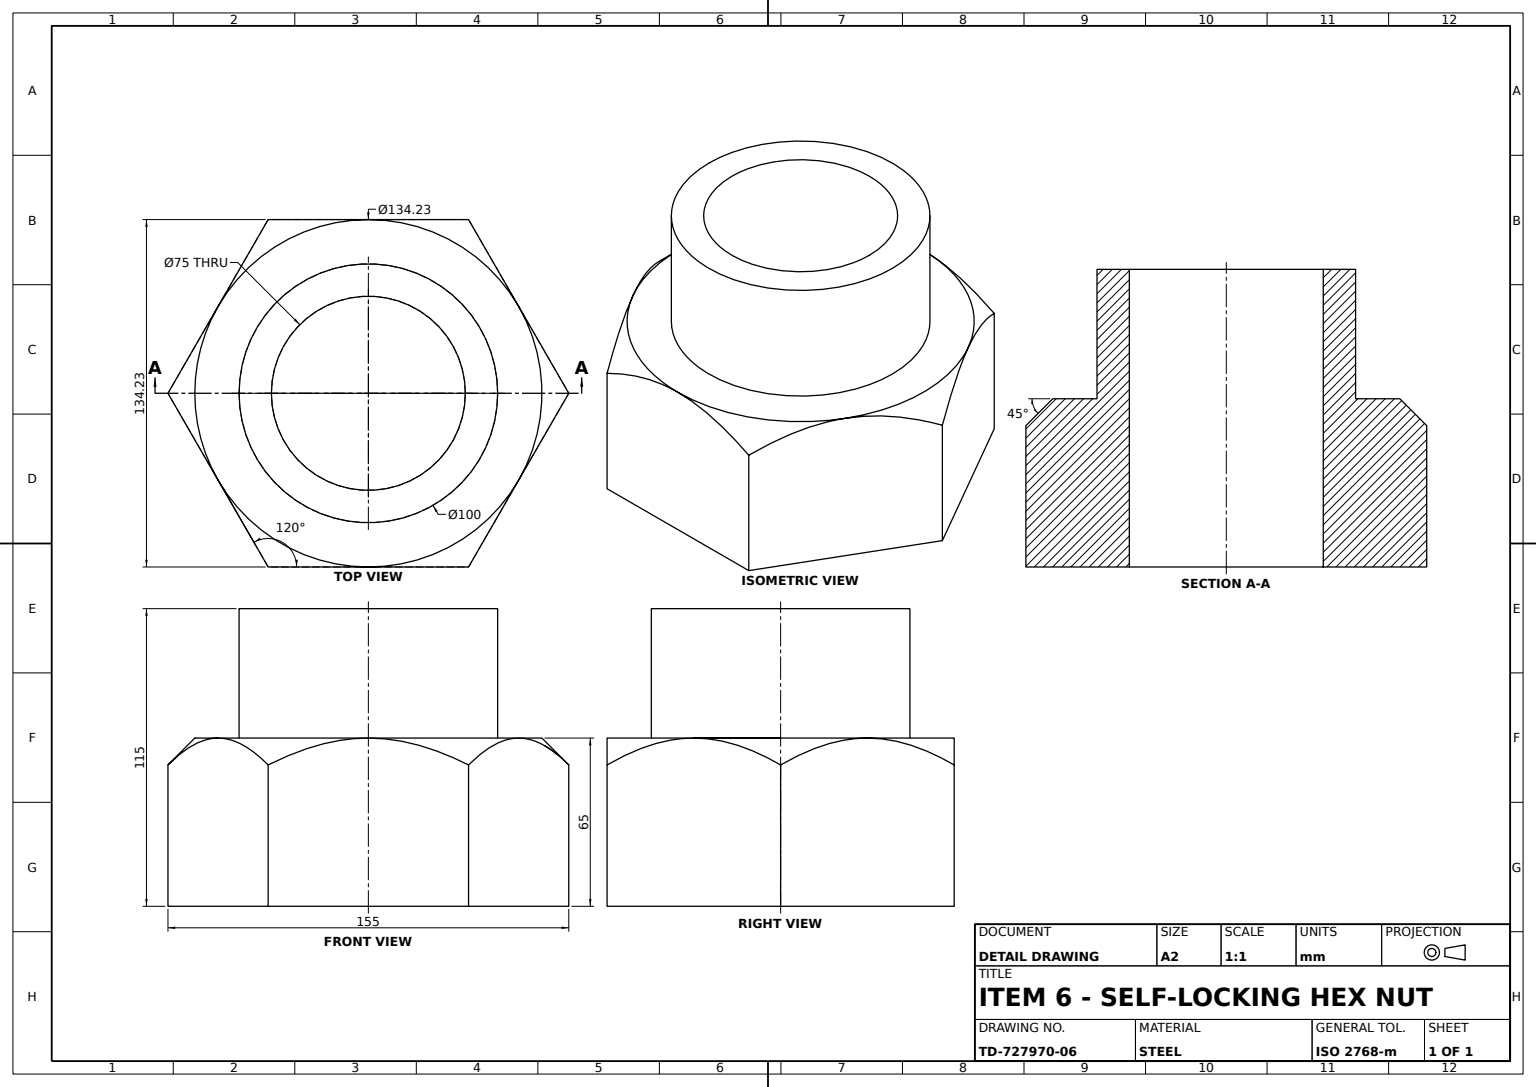
ISO-10303-21;
HEADER;
FILE_DESCRIPTION((''),'2;1');
FILE_NAME('','',(''),(''),'','','');
FILE_SCHEMA(('AUTOMOTIVE_DESIGN'));
ENDSEC;
DATA;
#1=APPLICATION_CONTEXT('');
#2=PRODUCT_CONTEXT('',#1,'mechanical');
#3=PRODUCT('','','',(#2));
#4=PRODUCT_DEFINITION_FORMATION('','',#3);
#5=PRODUCT_DEFINITION_CONTEXT('',#1,'design');
#6=PRODUCT_DEFINITION('','',#4,#5);
#7=PRODUCT_DEFINITION_SHAPE('','',#6);
#8=(LENGTH_UNIT()NAMED_UNIT(*)SI_UNIT(.MILLI.,.METRE.));
#9=(NAMED_UNIT(*)PLANE_ANGLE_UNIT()SI_UNIT($,.RADIAN.));
#10=(NAMED_UNIT(*)SI_UNIT($,.STERADIAN.)SOLID_ANGLE_UNIT());
#11=UNCERTAINTY_MEASURE_WITH_UNIT(LENGTH_MEASURE(1.E-05),#8,'distance_accuracy_value','');
#12=(GEOMETRIC_REPRESENTATION_CONTEXT(3)GLOBAL_UNCERTAINTY_ASSIGNED_CONTEXT((#11))GLOBAL_UNIT_ASSIGNED_CONTEXT((#8,#9,#10))REPRESENTATION_CONTEXT('',''));
#13=CARTESIAN_POINT('',(67.116969,54.616969,38.75));
#14=VERTEX_POINT('',#13);
#15=CARTESIAN_POINT('',(67.116969,0.,38.75));
#16=VERTEX_POINT('',#15);
#17=CARTESIAN_POINT('',(67.116969,65.,38.75));
#18=DIRECTION('',(0.,-1.,0.));
#19=VECTOR('',#18,1000.);
#20=LINE('',#17,#19);
#21=EDGE_CURVE('',#14,#16,#20,.T.);
#22=ORIENTED_EDGE('',*,*,#21,.F.);
#23=CARTESIAN_POINT('',(33.558484,65.,58.125));
#24=VERTEX_POINT('',#23);
#25=CARTESIAN_POINT('',(36.477067,65.,56.439955));
#26=CARTESIAN_POINT('',(39.371091,64.744995,54.76909));
#27=CARTESIAN_POINT('',(45.113889,63.765152,51.453484));
#28=CARTESIAN_POINT('',(47.962709,63.040779,49.808717));
#29=CARTESIAN_POINT('',(52.206431,61.647853,47.358603));
#30=CARTESIAN_POINT('',(53.606862,61.135616,46.550064));
#31=CARTESIAN_POINT('',(56.376991,60.028957,44.950729));
#32=CARTESIAN_POINT('',(57.747736,59.434192,44.159329));
#33=CARTESIAN_POINT('',(61.822347,57.541035,41.806851));
#34=CARTESIAN_POINT('',(64.488787,56.13435,40.267382));
#35=B_SPLINE_CURVE_WITH_KNOTS('',3,(#23,#25,#26,#27,#28,#29,#30,#31,#32,#33,#34,#13),.UNSPECIFIED.,.F.,.F.,(4,2,2,2,2,4),(0.040168143,0.050139784,0.060111425,0.065097246,0.070083066,0.080054708),.UNSPECIFIED.);
#36=EDGE_CURVE('',#24,#14,#35,.T.);
#37=ORIENTED_EDGE('',*,*,#36,.F.);
#38=CARTESIAN_POINT('',(0.,54.616969,77.5));
#39=VERTEX_POINT('',#38);
#40=CARTESIAN_POINT('',(2.63123,56.13611,75.980859));
#41=CARTESIAN_POINT('',(5.292688,57.539382,74.444265));
#42=CARTESIAN_POINT('',(10.692825,60.049913,71.326495));
#43=CARTESIAN_POINT('',(13.431518,61.157119,69.74531));
#44=CARTESIAN_POINT('',(19.006515,62.99736,66.526583));
#45=CARTESIAN_POINT('',(21.842887,63.730137,64.889003));
#46=CARTESIAN_POINT('',(26.187852,64.482743,62.380436));
#47=CARTESIAN_POINT('',(27.651256,64.6758,61.53554));
#48=CARTESIAN_POINT('',(30.611074,64.935371,59.826688));
#49=CARTESIAN_POINT('',(32.0889,65.,58.973465));
#50=B_SPLINE_CURVE_WITH_KNOTS('',3,(#38,#40,#41,#42,#43,#44,#45,#46,#47,#48,#49,#23),.UNSPECIFIED.,.F.,.F.,(4,2,2,2,2,4),(0.000000254,0.010042227,0.020084199,0.030126171,0.035147157,0.040168143),.UNSPECIFIED.);
#51=EDGE_CURVE('',#39,#24,#50,.T.);
#52=ORIENTED_EDGE('',*,*,#51,.F.);
#53=CARTESIAN_POINT('',(0.,0.,77.5));
#54=VERTEX_POINT('',#53);
#55=CARTESIAN_POINT('',(0.,65.,77.5));
#56=LINE('',#55,#19);
#57=EDGE_CURVE('',#39,#54,#56,.T.);
#58=ORIENTED_EDGE('',*,*,#57,.T.);
#59=DIRECTION('',(0.866025404,0.,-0.5));
#60=VECTOR('',#59,1000.);
#61=LINE('',#53,#60);
#62=EDGE_CURVE('',#54,#16,#61,.T.);
#63=ORIENTED_EDGE('',*,*,#62,.T.);
#64=EDGE_LOOP('',(#22,#37,#52,#58,#63));
#65=FACE_OUTER_BOUND('',#64,.T.);
#66=DIRECTION('',(-0.5,0.,-0.866025404));
#67=DIRECTION('',(-0.866025404,0.,0.5));
#68=AXIS2_PLACEMENT_3D('',#55,#66,#67);
#69=PLANE('',#68);
#70=ADVANCED_FACE('',(#65),#69,.F.);
#71=CARTESIAN_POINT('',(33.558484,65.,-58.125));
#72=VERTEX_POINT('',#71);
#73=CARTESIAN_POINT('',(0.,54.616969,-77.5));
#74=VERTEX_POINT('',#73);
#75=CARTESIAN_POINT('',(30.639901,65.,-59.810045));
#76=CARTESIAN_POINT('',(27.745878,64.744995,-61.48091));
#77=CARTESIAN_POINT('',(22.003079,63.765152,-64.796516));
#78=CARTESIAN_POINT('',(19.15426,63.040779,-66.441283));
#79=CARTESIAN_POINT('',(14.910537,61.647853,-68.891397));
#80=CARTESIAN_POINT('',(13.510107,61.135616,-69.699936));
#81=CARTESIAN_POINT('',(10.739977,60.028957,-71.299271));
#82=CARTESIAN_POINT('',(9.369232,59.434192,-72.090671));
#83=CARTESIAN_POINT('',(5.294622,57.541035,-74.443149));
#84=CARTESIAN_POINT('',(2.628182,56.13435,-75.982618));
#85=B_SPLINE_CURVE_WITH_KNOTS('',3,(#71,#75,#76,#77,#78,#79,#80,#81,#82,#83,#84,#73),.UNSPECIFIED.,.F.,.F.,(4,2,2,2,2,4),(0.040168143,0.050139784,0.060111425,0.065097246,0.070083066,0.080054708),.UNSPECIFIED.);
#86=EDGE_CURVE('',#72,#74,#85,.T.);
#87=ORIENTED_EDGE('',*,*,#86,.T.);
#88=CARTESIAN_POINT('',(-33.558484,65.,-58.125));
#89=VERTEX_POINT('',#88);
#90=CARTESIAN_POINT('',(-2.63123,56.13611,-75.980859));
#91=CARTESIAN_POINT('',(-5.292688,57.539382,-74.444265));
#92=CARTESIAN_POINT('',(-10.692825,60.049913,-71.326495));
#93=CARTESIAN_POINT('',(-13.431518,61.157119,-69.74531));
#94=CARTESIAN_POINT('',(-19.006515,62.99736,-66.526583));
#95=CARTESIAN_POINT('',(-21.842887,63.730137,-64.889003));
#96=CARTESIAN_POINT('',(-26.187852,64.482743,-62.380436));
#97=CARTESIAN_POINT('',(-27.651256,64.6758,-61.53554));
#98=CARTESIAN_POINT('',(-30.611074,64.935371,-59.826688));
#99=CARTESIAN_POINT('',(-32.0889,65.,-58.973465));
#100=B_SPLINE_CURVE_WITH_KNOTS('',3,(#73,#90,#91,#92,#93,#94,#95,#96,#97,#98,#99,#88),.UNSPECIFIED.,.F.,.F.,(4,2,2,2,2,4),(0.000000254,0.010042227,0.020084199,0.030126171,0.035147157,0.040168143),.UNSPECIFIED.);
#101=EDGE_CURVE('',#74,#89,#100,.T.);
#102=ORIENTED_EDGE('',*,*,#101,.T.);
#103=CARTESIAN_POINT('',(0.,65.,0.));
#104=DIRECTION('',(0.,1.,0.));
#105=DIRECTION('',(0.,0.,1.));
#106=AXIS2_PLACEMENT_3D('',#103,#104,#105);
#107=CIRCLE('',#106,67.116969);
#108=EDGE_CURVE('',#72,#89,#107,.T.);
#109=ORIENTED_EDGE('',*,*,#108,.F.);
#110=EDGE_LOOP('',(#87,#102,#109));
#111=FACE_OUTER_BOUND('',#110,.T.);
#112=AXIS2_PLACEMENT_3D('',#103,#18,#105);
#113=CONICAL_SURFACE('',#112,67.116968793,0.785398163);
#114=ADVANCED_FACE('',(#111),#113,.T.);
#115=CARTESIAN_POINT('',(0.,115.,50.));
#116=VERTEX_POINT('',#115);
#117=CARTESIAN_POINT('',(0.,65.,50.));
#118=VERTEX_POINT('',#117);
#119=LINE('',#115,#19);
#120=EDGE_CURVE('',#116,#118,#119,.T.);
#121=ORIENTED_EDGE('',*,*,#120,.F.);
#122=CARTESIAN_POINT('',(0.,115.,-50.));
#123=VERTEX_POINT('',#122);
#124=CARTESIAN_POINT('',(0.,115.,0.));
#125=AXIS2_PLACEMENT_3D('',#124,#104,#105);
#126=CIRCLE('',#125,50.);
#127=EDGE_CURVE('',#123,#116,#126,.T.);
#128=ORIENTED_EDGE('',*,*,#127,.F.);
#129=CARTESIAN_POINT('',(0.,65.,-50.));
#130=VERTEX_POINT('',#129);
#131=LINE('',#122,#19);
#132=EDGE_CURVE('',#123,#130,#131,.T.);
#133=ORIENTED_EDGE('',*,*,#132,.T.);
#134=CIRCLE('',#106,50.);
#135=EDGE_CURVE('',#130,#118,#134,.T.);
#136=ORIENTED_EDGE('',*,*,#135,.T.);
#137=EDGE_LOOP('',(#121,#128,#133,#136));
#138=FACE_OUTER_BOUND('',#137,.T.);
#139=DIRECTION('',(0.,0.,-1.));
#140=AXIS2_PLACEMENT_3D('',#124,#18,#139);
#141=CYLINDRICAL_SURFACE('',#140,50.);
#142=ADVANCED_FACE('',(#138),#141,.T.);
#143=CARTESIAN_POINT('',(67.116969,65.,0.));
#144=VERTEX_POINT('',#143);
#145=EDGE_CURVE('',#144,#72,#107,.T.);
#146=ORIENTED_EDGE('',*,*,#145,.F.);
#147=CARTESIAN_POINT('',(67.116969,54.616969,-38.75));
#148=VERTEX_POINT('',#147);
#149=CARTESIAN_POINT('',(67.116969,65.,-3.36094));
#150=CARTESIAN_POINT('',(67.116969,64.746151,-6.726161));
#151=CARTESIAN_POINT('',(67.116969,64.11968,-10.9379));
#152=CARTESIAN_POINT('',(67.116969,63.979196,-11.77886));
#153=CARTESIAN_POINT('',(67.116969,63.67085,-13.448297));
#154=CARTESIAN_POINT('',(67.116969,63.502775,-14.27826));
#155=CARTESIAN_POINT('',(67.116969,62.959093,-16.754655));
#156=CARTESIAN_POINT('',(67.116969,62.544056,-18.387599));
#157=CARTESIAN_POINT('',(67.116969,61.158489,-23.238394));
#158=CARTESIAN_POINT('',(67.116969,60.048016,-26.408379));
#159=CARTESIAN_POINT('',(67.116969,57.5351,-32.648487));
#160=CARTESIAN_POINT('',(67.116969,56.132663,-35.718612));
#161=B_SPLINE_CURVE_WITH_KNOTS('',3,(#143,#149,#150,#151,#152,#153,#154,#155,#156,#157,#158,#159,#160,#147),.UNSPECIFIED.,.F.,.F.,(4,2,2,2,2,2,4),(0.166041946,0.176166652,0.178697828,0.181229005,0.186291358,0.196416063,0.206540769),.UNSPECIFIED.);
#162=EDGE_CURVE('',#144,#148,#161,.T.);
#163=ORIENTED_EDGE('',*,*,#162,.T.);
#164=CARTESIAN_POINT('',(64.485739,56.13611,-40.269141));
#165=CARTESIAN_POINT('',(61.824281,57.539382,-41.805735));
#166=CARTESIAN_POINT('',(56.424144,60.049913,-44.923505));
#167=CARTESIAN_POINT('',(53.685451,61.157119,-46.50469));
#168=CARTESIAN_POINT('',(48.110454,62.99736,-49.723417));
#169=CARTESIAN_POINT('',(45.274082,63.730137,-51.360997));
#170=CARTESIAN_POINT('',(40.929116,64.482743,-53.869564));
#171=CARTESIAN_POINT('',(39.465713,64.6758,-54.71446));
#172=CARTESIAN_POINT('',(36.505895,64.935371,-56.423312));
#173=CARTESIAN_POINT('',(35.028068,65.,-57.276535));
#174=B_SPLINE_CURVE_WITH_KNOTS('',3,(#147,#164,#165,#166,#167,#168,#169,#170,#171,#172,#173,#71),.UNSPECIFIED.,.F.,.F.,(4,2,2,2,2,4),(0.000000254,0.010042227,0.020084199,0.030126171,0.035147157,0.040168143),.UNSPECIFIED.);
#175=EDGE_CURVE('',#148,#72,#174,.T.);
#176=ORIENTED_EDGE('',*,*,#175,.T.);
#177=EDGE_LOOP('',(#146,#163,#176));
#178=FACE_OUTER_BOUND('',#177,.T.);
#179=ADVANCED_FACE('',(#178),#113,.T.);
#180=CARTESIAN_POINT('',(0.,0.,-77.5));
#181=VERTEX_POINT('',#180);
#182=CARTESIAN_POINT('',(0.,65.,-77.5));
#183=LINE('',#182,#19);
#184=EDGE_CURVE('',#74,#181,#183,.T.);
#185=ORIENTED_EDGE('',*,*,#184,.T.);
#186=CARTESIAN_POINT('',(-67.116969,0.,-38.75));
#187=VERTEX_POINT('',#186);
#188=VECTOR('',#67,1000.);
#189=LINE('',#180,#188);
#190=EDGE_CURVE('',#181,#187,#189,.T.);
#191=ORIENTED_EDGE('',*,*,#190,.T.);
#192=CARTESIAN_POINT('',(-67.116969,54.616969,-38.75));
#193=VERTEX_POINT('',#192);
#194=CARTESIAN_POINT('',(-67.116969,65.,-38.75));
#195=LINE('',#194,#19);
#196=EDGE_CURVE('',#193,#187,#195,.T.);
#197=ORIENTED_EDGE('',*,*,#196,.F.);
#198=CARTESIAN_POINT('',(-36.477067,65.,-56.439955));
#199=CARTESIAN_POINT('',(-39.371091,64.744995,-54.76909));
#200=CARTESIAN_POINT('',(-45.113889,63.765152,-51.453484));
#201=CARTESIAN_POINT('',(-47.962709,63.040779,-49.808717));
#202=CARTESIAN_POINT('',(-52.206431,61.647853,-47.358603));
#203=CARTESIAN_POINT('',(-53.606862,61.135616,-46.550064));
#204=CARTESIAN_POINT('',(-56.376991,60.028957,-44.950729));
#205=CARTESIAN_POINT('',(-57.747736,59.434192,-44.159329));
#206=CARTESIAN_POINT('',(-61.822347,57.541035,-41.806851));
#207=CARTESIAN_POINT('',(-64.488787,56.13435,-40.267382));
#208=B_SPLINE_CURVE_WITH_KNOTS('',3,(#88,#198,#199,#200,#201,#202,#203,#204,#205,#206,#207,#192),.UNSPECIFIED.,.F.,.F.,(4,2,2,2,2,4),(0.040168143,0.050139784,0.060111425,0.065097246,0.070083066,0.080054708),.UNSPECIFIED.);
#209=EDGE_CURVE('',#89,#193,#208,.T.);
#210=ORIENTED_EDGE('',*,*,#209,.F.);
#211=ORIENTED_EDGE('',*,*,#101,.F.);
#212=EDGE_LOOP('',(#185,#191,#197,#210,#211));
#213=FACE_OUTER_BOUND('',#212,.T.);
#214=DIRECTION('',(0.5,0.,0.866025404));
#215=AXIS2_PLACEMENT_3D('',#182,#214,#59);
#216=PLANE('',#215);
#217=ADVANCED_FACE('',(#213),#216,.F.);
#218=CARTESIAN_POINT('',(-33.558484,65.,58.125));
#219=VERTEX_POINT('',#218);
#220=CARTESIAN_POINT('',(0.,65.,67.116969));
#221=VERTEX_POINT('',#220);
#222=EDGE_CURVE('',#219,#221,#107,.T.);
#223=ORIENTED_EDGE('',*,*,#222,.F.);
#224=CARTESIAN_POINT('',(-30.639901,65.,59.810045));
#225=CARTESIAN_POINT('',(-27.745878,64.744995,61.48091));
#226=CARTESIAN_POINT('',(-22.003079,63.765152,64.796516));
#227=CARTESIAN_POINT('',(-19.15426,63.040779,66.441283));
#228=CARTESIAN_POINT('',(-14.910537,61.647853,68.891397));
#229=CARTESIAN_POINT('',(-13.510107,61.135616,69.699936));
#230=CARTESIAN_POINT('',(-10.739977,60.028957,71.299271));
#231=CARTESIAN_POINT('',(-9.369232,59.434192,72.090671));
#232=CARTESIAN_POINT('',(-5.294622,57.541035,74.443149));
#233=CARTESIAN_POINT('',(-2.628182,56.13435,75.982618));
#234=B_SPLINE_CURVE_WITH_KNOTS('',3,(#218,#224,#225,#226,#227,#228,#229,#230,#231,#232,#233,#38),.UNSPECIFIED.,.F.,.F.,(4,2,2,2,2,4),(0.040168143,0.050139784,0.060111425,0.065097246,0.070083066,0.080054708),.UNSPECIFIED.);
#235=EDGE_CURVE('',#219,#39,#234,.T.);
#236=ORIENTED_EDGE('',*,*,#235,.T.);
#237=DIRECTION('',(0.,-0.707106781,0.707106781));
#238=VECTOR('',#237,1000.);
#239=LINE('',#220,#238);
#240=EDGE_CURVE('',#221,#39,#239,.T.);
#241=ORIENTED_EDGE('',*,*,#240,.F.);
#242=EDGE_LOOP('',(#223,#236,#241));
#243=FACE_OUTER_BOUND('',#242,.T.);
#244=ADVANCED_FACE('',(#243),#113,.T.);
#245=CARTESIAN_POINT('',(67.116969,56.13273,35.718477));
#246=CARTESIAN_POINT('',(67.116969,57.535933,32.646863));
#247=CARTESIAN_POINT('',(67.116969,60.051231,26.39995));
#248=CARTESIAN_POINT('',(67.116969,61.163337,23.224654));
#249=CARTESIAN_POINT('',(67.116969,62.550962,18.361792));
#250=CARTESIAN_POINT('',(67.116969,62.966611,16.724136));
#251=CARTESIAN_POINT('',(67.116969,63.692297,13.411207));
#252=CARTESIAN_POINT('',(67.116969,64.002385,11.732462));
#253=CARTESIAN_POINT('',(67.116969,64.7468,6.709607));
#254=CARTESIAN_POINT('',(67.116969,65.,3.356938));
#255=B_SPLINE_CURVE_WITH_KNOTS('',3,(#13,#245,#246,#247,#248,#249,#250,#251,#252,#253,#254,#143),.UNSPECIFIED.,.F.,.F.,(4,2,2,2,2,4),(0.125591343,0.135703994,0.145816645,0.15087297,0.155929296,0.166041946),.UNSPECIFIED.);
#256=EDGE_CURVE('',#14,#144,#255,.T.);
#257=ORIENTED_EDGE('',*,*,#256,.T.);
#258=EDGE_CURVE('',#24,#144,#107,.T.);
#259=ORIENTED_EDGE('',*,*,#258,.F.);
#260=ORIENTED_EDGE('',*,*,#36,.T.);
#261=EDGE_LOOP('',(#257,#259,#260));
#262=FACE_OUTER_BOUND('',#261,.T.);
#263=ADVANCED_FACE('',(#262),#113,.T.);
#264=CARTESIAN_POINT('',(-67.116969,54.616969,38.75));
#265=VERTEX_POINT('',#264);
#266=CARTESIAN_POINT('',(-64.485739,56.13611,40.269141));
#267=CARTESIAN_POINT('',(-61.824281,57.539382,41.805735));
#268=CARTESIAN_POINT('',(-56.424144,60.049913,44.923505));
#269=CARTESIAN_POINT('',(-53.685451,61.157119,46.50469));
#270=CARTESIAN_POINT('',(-48.110454,62.99736,49.723417));
#271=CARTESIAN_POINT('',(-45.274082,63.730137,51.360997));
#272=CARTESIAN_POINT('',(-40.929116,64.482743,53.869564));
#273=CARTESIAN_POINT('',(-39.465713,64.6758,54.71446));
#274=CARTESIAN_POINT('',(-36.505895,64.935371,56.423312));
#275=CARTESIAN_POINT('',(-35.028068,65.,57.276535));
#276=B_SPLINE_CURVE_WITH_KNOTS('',3,(#264,#266,#267,#268,#269,#270,#271,#272,#273,#274,#275,#218),.UNSPECIFIED.,.F.,.F.,(4,2,2,2,2,4),(0.000000254,0.010042227,0.020084199,0.030126171,0.035147157,0.040168143),.UNSPECIFIED.);
#277=EDGE_CURVE('',#265,#219,#276,.T.);
#278=ORIENTED_EDGE('',*,*,#277,.T.);
#279=CARTESIAN_POINT('',(-67.116969,65.,0.));
#280=VERTEX_POINT('',#279);
#281=EDGE_CURVE('',#280,#219,#107,.T.);
#282=ORIENTED_EDGE('',*,*,#281,.F.);
#283=CARTESIAN_POINT('',(-67.116969,65.,3.36094));
#284=CARTESIAN_POINT('',(-67.116969,64.746151,6.726161));
#285=CARTESIAN_POINT('',(-67.116969,64.11968,10.9379));
#286=CARTESIAN_POINT('',(-67.116969,63.979196,11.77886));
#287=CARTESIAN_POINT('',(-67.116969,63.67085,13.448297));
#288=CARTESIAN_POINT('',(-67.116969,63.502775,14.27826));
#289=CARTESIAN_POINT('',(-67.116969,62.959093,16.754655));
#290=CARTESIAN_POINT('',(-67.116969,62.544056,18.387599));
#291=CARTESIAN_POINT('',(-67.116969,61.158489,23.238394));
#292=CARTESIAN_POINT('',(-67.116969,60.048016,26.408379));
#293=CARTESIAN_POINT('',(-67.116969,57.5351,32.648487));
#294=CARTESIAN_POINT('',(-67.116969,56.132663,35.718612));
#295=B_SPLINE_CURVE_WITH_KNOTS('',3,(#279,#283,#284,#285,#286,#287,#288,#289,#290,#291,#292,#293,#294,#264),.UNSPECIFIED.,.F.,.F.,(4,2,2,2,2,2,4),(0.166041946,0.176166652,0.178697828,0.181229005,0.186291358,0.196416063,0.206540769),.UNSPECIFIED.);
#296=EDGE_CURVE('',#280,#265,#295,.T.);
#297=ORIENTED_EDGE('',*,*,#296,.T.);
#298=EDGE_LOOP('',(#278,#282,#297));
#299=FACE_OUTER_BOUND('',#298,.T.);
#300=ADVANCED_FACE('',(#299),#113,.T.);
#301=ORIENTED_EDGE('',*,*,#62,.F.);
#302=CARTESIAN_POINT('',(-67.116969,0.,38.75));
#303=VERTEX_POINT('',#302);
#304=DIRECTION('',(0.866025404,0.,0.5));
#305=VECTOR('',#304,1000.);
#306=LINE('',#302,#305);
#307=EDGE_CURVE('',#303,#54,#306,.T.);
#308=ORIENTED_EDGE('',*,*,#307,.F.);
#309=VECTOR('',#105,1000.);
#310=LINE('',#186,#309);
#311=EDGE_CURVE('',#187,#303,#310,.T.);
#312=ORIENTED_EDGE('',*,*,#311,.F.);
#313=ORIENTED_EDGE('',*,*,#190,.F.);
#314=CARTESIAN_POINT('',(67.116969,0.,-38.75));
#315=VERTEX_POINT('',#314);
#316=DIRECTION('',(-0.866025404,0.,-0.5));
#317=VECTOR('',#316,1000.);
#318=LINE('',#314,#317);
#319=EDGE_CURVE('',#315,#181,#318,.T.);
#320=ORIENTED_EDGE('',*,*,#319,.F.);
#321=VECTOR('',#139,1000.);
#322=LINE('',#15,#321);
#323=EDGE_CURVE('',#16,#315,#322,.T.);
#324=ORIENTED_EDGE('',*,*,#323,.F.);
#325=EDGE_LOOP('',(#301,#308,#312,#313,#320,#324));
#326=FACE_OUTER_BOUND('',#325,.T.);
#327=CARTESIAN_POINT('',(0.,0.,37.5));
#328=VERTEX_POINT('',#327);
#329=CARTESIAN_POINT('',(0.,0.,-37.5));
#330=VERTEX_POINT('',#329);
#331=CARTESIAN_POINT('',(0.,0.,0.));
#332=AXIS2_PLACEMENT_3D('',#331,#104,#105);
#333=CIRCLE('',#332,37.5);
#334=EDGE_CURVE('',#328,#330,#333,.T.);
#335=ORIENTED_EDGE('',*,*,#334,.T.);
#336=EDGE_CURVE('',#330,#328,#333,.T.);
#337=ORIENTED_EDGE('',*,*,#336,.T.);
#338=EDGE_LOOP('',(#335,#337));
#339=FACE_BOUND('',#338,.T.);
#340=PLANE('',#332);
#341=ADVANCED_FACE('',(#326,#339),#340,.F.);
#342=ORIENTED_EDGE('',*,*,#196,.T.);
#343=ORIENTED_EDGE('',*,*,#311,.T.);
#344=CARTESIAN_POINT('',(-67.116969,65.,38.75));
#345=LINE('',#344,#19);
#346=EDGE_CURVE('',#265,#303,#345,.T.);
#347=ORIENTED_EDGE('',*,*,#346,.F.);
#348=ORIENTED_EDGE('',*,*,#296,.F.);
#349=CARTESIAN_POINT('',(-67.116969,56.13273,-35.718477));
#350=CARTESIAN_POINT('',(-67.116969,57.535933,-32.646863));
#351=CARTESIAN_POINT('',(-67.116969,60.051231,-26.39995));
#352=CARTESIAN_POINT('',(-67.116969,61.163337,-23.224654));
#353=CARTESIAN_POINT('',(-67.116969,62.550962,-18.361792));
#354=CARTESIAN_POINT('',(-67.116969,62.966611,-16.724136));
#355=CARTESIAN_POINT('',(-67.116969,63.692297,-13.411207));
#356=CARTESIAN_POINT('',(-67.116969,64.002385,-11.732462));
#357=CARTESIAN_POINT('',(-67.116969,64.7468,-6.709607));
#358=CARTESIAN_POINT('',(-67.116969,65.,-3.356938));
#359=B_SPLINE_CURVE_WITH_KNOTS('',3,(#192,#349,#350,#351,#352,#353,#354,#355,#356,#357,#358,#279),.UNSPECIFIED.,.F.,.F.,(4,2,2,2,2,4),(0.125591343,0.135703994,0.145816645,0.15087297,0.155929296,0.166041946),.UNSPECIFIED.);
#360=EDGE_CURVE('',#193,#280,#359,.T.);
#361=ORIENTED_EDGE('',*,*,#360,.F.);
#362=EDGE_LOOP('',(#342,#343,#347,#348,#361));
#363=FACE_OUTER_BOUND('',#362,.T.);
#364=DIRECTION('',(1.,0.,0.));
#365=AXIS2_PLACEMENT_3D('',#194,#364,#139);
#366=PLANE('',#365);
#367=ADVANCED_FACE('',(#363),#366,.F.);
#368=ORIENTED_EDGE('',*,*,#184,.F.);
#369=ORIENTED_EDGE('',*,*,#86,.F.);
#370=ORIENTED_EDGE('',*,*,#175,.F.);
#371=CARTESIAN_POINT('',(67.116969,65.,-38.75));
#372=LINE('',#371,#19);
#373=EDGE_CURVE('',#148,#315,#372,.T.);
#374=ORIENTED_EDGE('',*,*,#373,.T.);
#375=ORIENTED_EDGE('',*,*,#319,.T.);
#376=EDGE_LOOP('',(#368,#369,#370,#374,#375));
#377=FACE_OUTER_BOUND('',#376,.T.);
#378=DIRECTION('',(-0.5,0.,0.866025404));
#379=AXIS2_PLACEMENT_3D('',#371,#378,#304);
#380=PLANE('',#379);
#381=ADVANCED_FACE('',(#377),#380,.F.);
#382=ORIENTED_EDGE('',*,*,#235,.F.);
#383=ORIENTED_EDGE('',*,*,#277,.F.);
#384=ORIENTED_EDGE('',*,*,#346,.T.);
#385=ORIENTED_EDGE('',*,*,#307,.T.);
#386=ORIENTED_EDGE('',*,*,#57,.F.);
#387=EDGE_LOOP('',(#382,#383,#384,#385,#386));
#388=FACE_OUTER_BOUND('',#387,.T.);
#389=DIRECTION('',(0.5,0.,-0.866025404));
#390=AXIS2_PLACEMENT_3D('',#344,#389,#316);
#391=PLANE('',#390);
#392=ADVANCED_FACE('',(#388),#391,.F.);
#393=CARTESIAN_POINT('',(0.,115.,-37.5));
#394=VERTEX_POINT('',#393);
#395=LINE('',#393,#19);
#396=EDGE_CURVE('',#394,#330,#395,.T.);
#397=ORIENTED_EDGE('',*,*,#396,.T.);
#398=ORIENTED_EDGE('',*,*,#334,.F.);
#399=CARTESIAN_POINT('',(0.,115.,37.5));
#400=VERTEX_POINT('',#399);
#401=LINE('',#399,#19);
#402=EDGE_CURVE('',#400,#328,#401,.T.);
#403=ORIENTED_EDGE('',*,*,#402,.F.);
#404=CIRCLE('',#125,37.5);
#405=EDGE_CURVE('',#400,#394,#404,.T.);
#406=ORIENTED_EDGE('',*,*,#405,.T.);
#407=EDGE_LOOP('',(#397,#398,#403,#406));
#408=FACE_OUTER_BOUND('',#407,.T.);
#409=CYLINDRICAL_SURFACE('',#140,37.5);
#410=ADVANCED_FACE('',(#408),#409,.F.);
#411=ORIENTED_EDGE('',*,*,#21,.T.);
#412=ORIENTED_EDGE('',*,*,#323,.T.);
#413=ORIENTED_EDGE('',*,*,#373,.F.);
#414=ORIENTED_EDGE('',*,*,#162,.F.);
#415=ORIENTED_EDGE('',*,*,#256,.F.);
#416=EDGE_LOOP('',(#411,#412,#413,#414,#415));
#417=FACE_OUTER_BOUND('',#416,.T.);
#418=DIRECTION('',(-1.,0.,0.));
#419=AXIS2_PLACEMENT_3D('',#17,#418,#105);
#420=PLANE('',#419);
#421=ADVANCED_FACE('',(#417),#420,.F.);
#422=ORIENTED_EDGE('',*,*,#209,.T.);
#423=ORIENTED_EDGE('',*,*,#360,.T.);
#424=EDGE_CURVE('',#89,#280,#107,.T.);
#425=ORIENTED_EDGE('',*,*,#424,.F.);
#426=EDGE_LOOP('',(#422,#423,#425));
#427=FACE_OUTER_BOUND('',#426,.T.);
#428=ADVANCED_FACE('',(#427),#113,.T.);
#429=ORIENTED_EDGE('',*,*,#135,.F.);
#430=EDGE_CURVE('',#118,#130,#134,.T.);
#431=ORIENTED_EDGE('',*,*,#430,.F.);
#432=EDGE_LOOP('',(#429,#431));
#433=FACE_BOUND('',#432,.T.);
#434=ORIENTED_EDGE('',*,*,#258,.T.);
#435=ORIENTED_EDGE('',*,*,#145,.T.);
#436=ORIENTED_EDGE('',*,*,#108,.T.);
#437=ORIENTED_EDGE('',*,*,#424,.T.);
#438=ORIENTED_EDGE('',*,*,#281,.T.);
#439=ORIENTED_EDGE('',*,*,#222,.T.);
#440=EDGE_CURVE('',#221,#24,#107,.T.);
#441=ORIENTED_EDGE('',*,*,#440,.T.);
#442=EDGE_LOOP('',(#434,#435,#436,#437,#438,#439,#441));
#443=FACE_OUTER_BOUND('',#442,.T.);
#444=PLANE('',#106);
#445=ADVANCED_FACE('',(#433,#443),#444,.T.);
#446=ORIENTED_EDGE('',*,*,#120,.T.);
#447=ORIENTED_EDGE('',*,*,#430,.T.);
#448=ORIENTED_EDGE('',*,*,#132,.F.);
#449=EDGE_CURVE('',#116,#123,#126,.T.);
#450=ORIENTED_EDGE('',*,*,#449,.F.);
#451=EDGE_LOOP('',(#446,#447,#448,#450));
#452=FACE_OUTER_BOUND('',#451,.T.);
#453=ADVANCED_FACE('',(#452),#141,.T.);
#454=ORIENTED_EDGE('',*,*,#240,.T.);
#455=ORIENTED_EDGE('',*,*,#51,.T.);
#456=ORIENTED_EDGE('',*,*,#440,.F.);
#457=EDGE_LOOP('',(#454,#455,#456));
#458=FACE_OUTER_BOUND('',#457,.T.);
#459=ADVANCED_FACE('',(#458),#113,.T.);
#460=ORIENTED_EDGE('',*,*,#402,.T.);
#461=ORIENTED_EDGE('',*,*,#336,.F.);
#462=ORIENTED_EDGE('',*,*,#396,.F.);
#463=EDGE_CURVE('',#394,#400,#404,.T.);
#464=ORIENTED_EDGE('',*,*,#463,.T.);
#465=EDGE_LOOP('',(#460,#461,#462,#464));
#466=FACE_OUTER_BOUND('',#465,.T.);
#467=ADVANCED_FACE('',(#466),#409,.F.);
#468=ORIENTED_EDGE('',*,*,#127,.T.);
#469=ORIENTED_EDGE('',*,*,#449,.T.);
#470=EDGE_LOOP('',(#468,#469));
#471=FACE_OUTER_BOUND('',#470,.T.);
#472=ORIENTED_EDGE('',*,*,#463,.F.);
#473=ORIENTED_EDGE('',*,*,#405,.F.);
#474=EDGE_LOOP('',(#472,#473));
#475=FACE_BOUND('',#474,.T.);
#476=PLANE('',#125);
#477=ADVANCED_FACE('',(#471,#475),#476,.T.);
#478=CLOSED_SHELL('',(#70,#114,#142,#179,#217,#244,#263,#300,#341,#367,#381,#392,#410,#421,#428,#445,#453,#459,#467,#477));
#479=MANIFOLD_SOLID_BREP('',#478);
#480=ADVANCED_BREP_SHAPE_REPRESENTATION('',(#479),#12);
#481=SHAPE_DEFINITION_REPRESENTATION(#7,#480);
ENDSEC;
END-ISO-10303-21;
